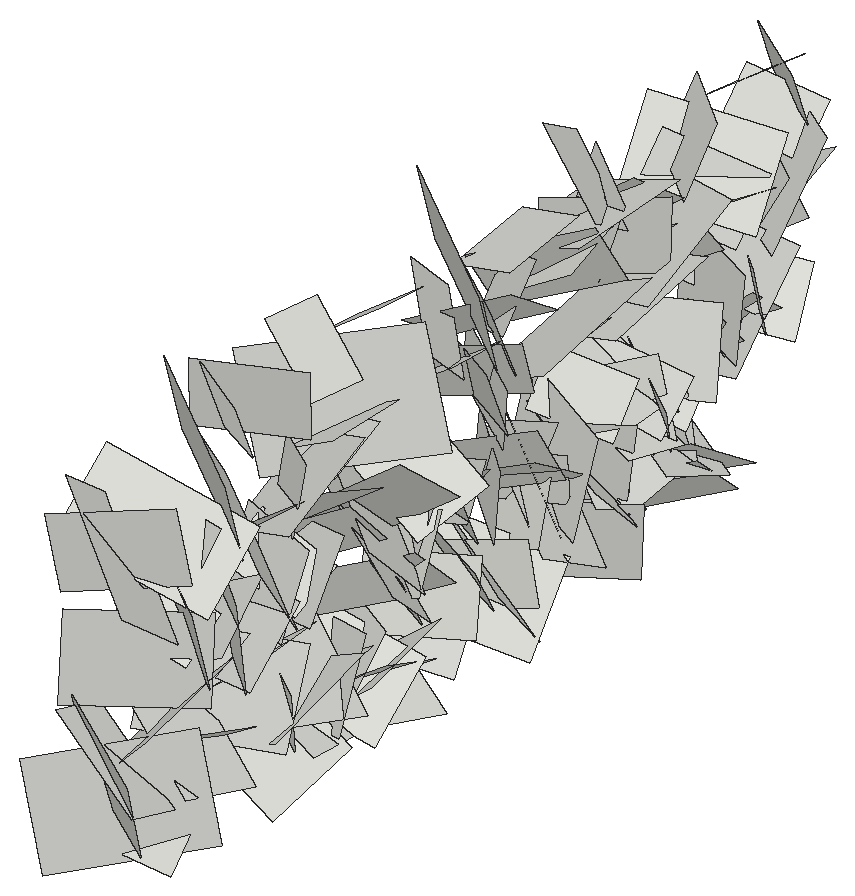
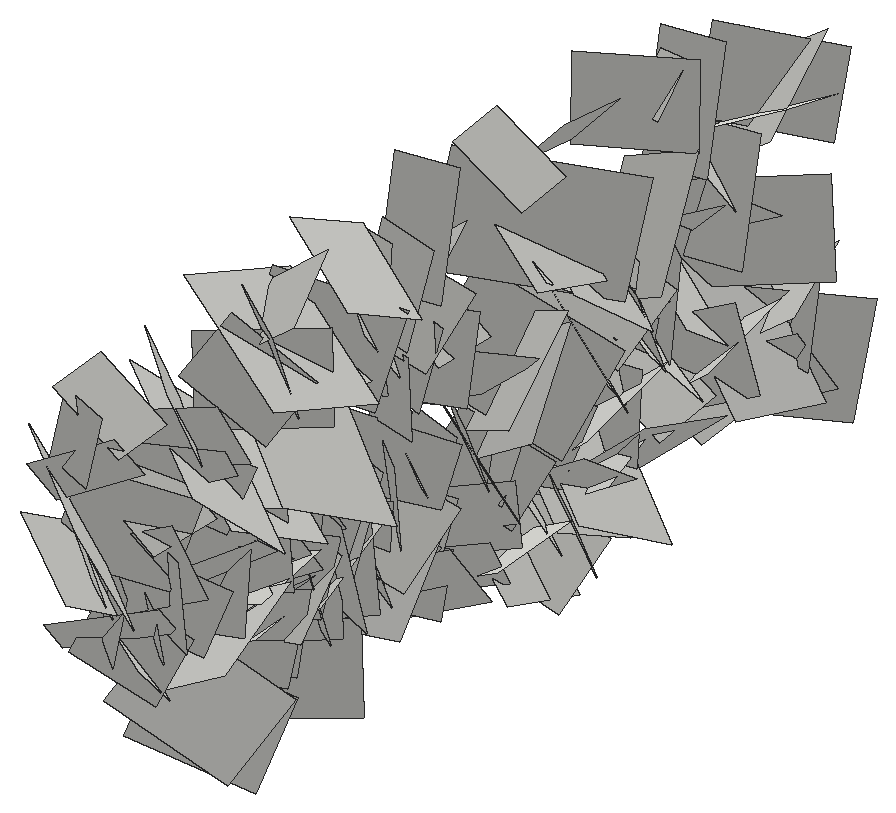
# SketchUp Ruby script. Lengths in inches.
U = 1.inch
M = Sketchup.active_model
def pt(a) = Geom::Point3d.new(a.map { |v| v * U })
def face(e, loops, mat)
  f = e.add_face(loops[0].map { |a| pt(a) })
  loops[1..].each { |l| e.add_face(l.map { |a| pt(a) }).erase! }
  f.material = f.back_material = mat if mat
  f
end
# faces: each face lists its corners as indices into pts; further lists are holes
def faces(e, pts, list, mat = nil) = list.each { |f| face(e, (f[0].is_a?(Array) ? f : [f]).map { |l| l.map { |i| pts[i] } }, mat) }
# xy, xz, yz: faces in a plane at the given z, y or x. An outline is a flat list of corners, or four numbers for a rectangle; further outlines are holes
def ring(l) = l.size == 4 ? [[l[0], l[1]], [l[2], l[1]], [l[2], l[3]], [l[0], l[3]]] : l.each_slice(2).to_a
def flat(e, list, mat, &to3) = list.each { |f| face(e, (f[0].is_a?(Array) ? f : [f]).map { |l| ring(l).map { |u, v| to3.(u, v) } }, mat) }
def xy(e, z, list, mat = nil) = flat(e, list, mat) { |x, y| [x, y, z] }
def xz(e, y, list, mat = nil) = flat(e, list, mat) { |x, z| [x, y, z] }
def yz(e, x, list, mat = nil) = flat(e, list, mat) { |y, z| [x, y, z] }
def lines(e, pts, list) = list.each { |a, b| e.add_line(pt(pts[a]), pt(pts[b])) }
# prism: a flat outline (further loops are holes) pulled along v
def prism(e, loops, v, mat = nil)
  f = face(e, loops, mat); d = Geom::Vector3d.new(v.map { |x| x * U })
  f.pushpull(f.normal.samedirection?(d) ? d.length : -d.length)
end
def box(e, o, s, mat = nil) = prism(e, [[o, [o[0] + s[0], o[1], o[2]], [o[0] + s[0], o[1] + s[1], o[2]], [o[0], o[1] + s[1], o[2]]]], [0, 0, s[2]], mat)
def at(x, y, z, deg = 0) = Geom::Transformation.translation(pt([x, y, z])) * Geom::Transformation.rotation(ORIGIN, Z_AXIS, deg.degrees)
def axes(o, x, y, z) = Geom::Transformation.new([*x, 0, *y, 0, *z, 0, *pt(o).to_a, 1])
def part(name) = M.definitions.add(name)
# library, detail: a bought-in or finely detailed component or shape, given as its bounding box
def library(name, o, s) = part(name).tap { |d| box(d.entities, o, s) }
def detail(e, o, s) = box(e.add_group.entities, o, s)
def put(e, d, t, mat = nil) = e.add_instance(d, t).tap { |i| i.material = mat if mat }
def group(e, t, mat = nil) = e.add_group.tap { |g| g.transformation = t; g.material = mat if mat }.entities
root = M.entities
c1 = part("Component\#6")
p = [[0.01,0,0],[0,3.24,4.54],[4.32,3.24,4.54],[4.33,0,0]]
faces(c1.entities,p,[[0,1,2,3]])
put(root,c1,axes([404.88,126.77,21.87],[0.10992,-0.34124,0.92241],[-0.05569,0.92428,0.34784],[-1.04103,-0.08548,0.07879]))
put(root,c1,axes([400.91,126.29,27.49],[-0.18614,0.86586,-0.34095],[-0.04817,-0.35453,-0.87695],[0.98523,0.14625,-0.10729]))
put(root,c1,axes([404.88,129.02,36.97],[0.03047,0.19902,-0.90037],[-0.05941,-0.89877,-0.20045],[-0.97562,0.06094,-0.01591]))
put(root,c1,axes([404.88,130.54,26.21],[0.16316,0.13144,-1.2549],[0.21583,-1.25022,-0.10597],[-1.31994,-0.18819,-0.17245]))
put(root,c1,axes([404.88,129.15,30.625],[0.089,-0.93417,0.70597],[0.20388,0.70917,0.91554],[-1.22433,0.05019,0.20378]))
put(root,c1,axes([404.88,131.26,22.93],[-0.10206,-0.4663,-0.72841],[-0.02316,-0.73136,0.47108],[-0.91647,0.07041,0.06921]))
put(root,c1,axes([404.88,131.58,31.0625],[-0.07279,0.01987,-1.05868],[0.10279,-1.05633,-0.02611],[-1.11768,-0.09844,0.06655]))
put(root,c1,axes([404.88,127.1,26.99],[0.01407,1.25738,0.35681],[0.29384,0.346,-1.2296],[-1.35392,0.08816,-0.26315]))
put(root,c1,axes([404.88,134.48,33.76],[0.26334,-1.11466,-0.41014],[-0.1173,-0.43892,1.12584],[-1.25351,-0.19309,-0.19152]))
put(root,c1,axes([400.91,129.75,30.06],[0.01937,0.49926,0.36665],[0.0577,0.36409,-0.4985],[0.65405,-0.04691,0.03312]))
put(root,c1,axes([404.88,131.21,27.63],[0.2234,-0.54463,1.08834],[0.02633,1.10624,0.54877],[-1.28976,-0.07175,0.19972]))
put(root,c1,axes([400.91,134.18,33.55],[-0.07538,-0.44425,-0.62436],[0.04133,-0.62833,0.44263],[0.8112,-0.00926,-0.08057]))
put(root,c1,axes([404.88,134.17,21.91],[0.00769,-1.04417,0.30366],[0.13881,0.30229,1.03635],[-1.14428,0.02965,0.12776]))
put(root,c1,axes([400.91,134.6875,22.2],[-0.10426,-0.66856,0.17597],[0.06243,0.169,0.67497],[0.73015,-0.10992,-0.03258]))
put(root,c1,axes([404.88,133.37,32.625],[0.2234,-0.54463,1.08834],[0.02633,1.10624,0.54877],[-1.28976,-0.07175,0.19972]))
put(root,c1,axes([404.88,131.97,28.78],[-0.10091,0.74431,0.53228],[0.01265,0.53611,-0.74754],[-0.96987,-0.07045,-0.06513]))
put(root,c1,axes([404.88,137.68,26.93],[-0.04018,-0.30696,-1.06119],[0.15368,-1.05402,0.2997],[-1.16085,-0.12891,0.07641]))
put(root,c1,axes([404.88,133.57,26.39],[0.0097,-0.16576,1.00827],[0.11893,1.00238,0.16377],[-1.07657,0.10924,0.02717]))
put(root,c1,axes([400.91,135.55,39.48],[0.03347,0.37514,-0.47819],[-0.05412,-0.47551,-0.37641],[0.64197,-0.05964,-0.0068]))
put(root,c1,axes([404.88,133.77,26.39],[0.09062,0.64279,0.71838],[-0.13606,0.72237,-0.63108],[-1.01272,-0.03954,0.14907]))
put(root,c1,axes([404.88,134.64,27.51],[-0.11331,0.92563,-0.03565],[0.09128,-0.0258,-0.92812],[-0.97764,-0.10969,-0.08252]))
put(root,c1,axes([404.88,136.8125,27.97],[0.23976,-0.84366,1.03424],[0.08712,1.0558,0.84327],[-1.41209,-0.07811,0.22763]))
put(root,c1,axes([404.88,137.68,39.44],[-0.12024,0.16456,-0.83242],[-0.12638,-0.83458,-0.14874],[-0.89051,0.09622,0.13351]))
put(root,c1,axes([404.88,140.34,20.98],[-0.05969,-1.08852,-0.33352],[0.17093,-0.33819,1.07653],[-1.19461,0.00599,0.1707]))
put(root,c1,axes([404.88,135.78,27.7],[0.08438,0.31612,0.89331],[-0.15155,0.8902,-0.30228],[-0.99295,-0.109,0.12205]))
put(root,c1,axes([400.91,138.35,27.1],[-0.19626,0.31166,-0.79897],[0.02742,-0.81497,-0.3239],[0.90864,0.09191,-0.1628]))
put(root,c1,axes([400.91,136.92,29.78],[0.03864,0.57092,0.32429],[-0.05823,0.3263,-0.56829],[0.69355,-0.00442,-0.06578]))
put(root,c1,axes([404.88,135.48,23.28],[0.21581,1.04519,0.5846],[0.09636,0.57779,-1.06467],[-1.26577,0.22219,0.01862]))
put(root,c1,axes([400.91,141.16,33.73],[0.01034,-0.20439,-0.70125],[-0.11317,-0.69418,0.20085],[0.76594,-0.09981,0.03914]))
put(root,c1,axes([400.91,137.77,24.11],[-0.1419,0.78136,-0.16109],[0.04598,-0.15597,-0.79258],[0.84441,0.13979,0.01609]))
put(root,c1,axes([404.88,141.41,21.99],[-0.04242,-1.10503,0.33762],[0.18816,0.32793,1.09436],[-1.21025,0.08972,0.15831]))
put(root,c1,axes([404.88,136.3,32.46],[0.17238,0.91042,0.71253],[0.07022,0.71102,-0.92361],[-1.22345,0.16908,0.04738]))
put(root,c1,axes([404.88,137.68,27.62],[-0.00267,0.49736,0.77514],[-0.05686,0.77375,-0.49665],[-0.97459,-0.04651,0.02685]))
put(root,c1,axes([404.88,138.75,33.42],[-0.07987,0.93748,-0.3836],[0.04246,-0.3816,-0.94046],[-1.07286,-0.0849,-0.00867]))
put(root,c1,axes([400.91,143.53,22.21],[-0.15224,-0.84766,-0.36991],[-0.10957,-0.35729,0.85887],[0.97421,-0.17265,0.03879]))
put(root,c1,axes([400.91,139.71,39.61],[0.08624,0.67106,-0.00672],[-0.16105,0.01183,-0.6586],[0.69289,-0.08077,-0.15225]))
put(root,c1,axes([404.88,139.49,21.74],[-0.04906,0.46783,0.90513],[-0.0041,0.90598,-0.46846],[-1.08001,-0.02469,-0.03934]))
put(root,c1,axes([400.91,142.28,27.34],[-0.09885,-0.42767,0.49172],[0.03253,0.4933,0.43487],[0.69002,-0.08452,0.04994]))
put(root,c1,axes([400.91,144.18,33.46],[-0.08879,-0.56105,-0.39599],[0.0694,-0.40364,0.55803],[0.72461,-0.03009,-0.10197]))
put(root,c1,axes([404.88,145.12,23.07],[0.0526,-0.82286,-0.58821],[-0.0059,-0.58914,0.82367],[-1.07215,-0.03713,-0.03339]))
put(root,c1,axes([400.91,144.73,33.27],[-0.16555,-0.76551,-0.15352],[0.02389,-0.16091,0.77946],[0.82725,-0.14855,-0.05323]))
put(root,c1,axes([400.91,142.8,24.59],[-0.06246,-0.31977,0.5346],[0.03506,0.53462,0.32343],[0.65938,-0.05871,0.03344]))
put(root,c1,axes([404.88,145.05,38.54],[0.26561,0.06521,-1.32838],[0.06869,-1.35074,-0.05408],[-1.4081,-0.05359,-0.25321]))
put(root,c1,axes([400.91,145.49,24.46],[-0.14807,-0.32942,-0.64401],[0.00647,-0.65643,0.33444],[0.76675,-0.05808,-0.12719]))
put(root,c1,axes([404.88,142.58,23.75],[-0.11698,0.88265,-0.34817],[0.00423,-0.35009,-0.88876],[-1.00576,-0.10414,0.03675]))
put(root,c1,axes([404.88,143.41,32.67],[0.00295,0.89075,-0.72818],[0.15415,-0.72261,-0.88339],[-1.20976,-0.08991,-0.11434]))
put(root,c1,axes([404.88,145.42,24.52],[0.2647,-0.88765,0.75819],[0.01358,0.77738,0.90589],[-1.23735,-0.18136,0.17214]))
put(root,c1,axes([404.88,141.63,23.18],[0.01995,1.00092,0.30572],[0.13829,0.30114,-0.99396],[-1.10071,0.05598,-0.11933]))
put(root,c1,axes([400.91,145.72,37.21],[0.0202,-0.65006,0.07365],[-0.02062,0.07308,0.65011],[0.69316,0.02112,0.01719]))
put(root,c1,axes([404.88,145.04,25.97],[0.0145,-0.85349,0.83598],[0.13626,0.83223,0.84756],[-1.25903,0.08024,0.10136]))
put(root,c1,axes([404.88,146.5,19.86],[-0.14062,-0.87102,0.18651],[-0.03259,0.19294,0.87915],[-0.94365,0.12313,-0.05815]))
put(root,c1,axes([400.91,145.6,27.28],[0.00806,0.29423,-0.56577],[0.12293,-0.55701,-0.28812],[0.6647,0.09945,0.06014]))
put(root,c1,axes([400.91,146.3,23.53],[-0.0913,-0.50535,0.50896],[0.05568,0.5068,0.51209],[0.75823,-0.09807,0.02368]))
put(root,c1,axes([404.88,144.65,25.96],[-0.15377,0.53431,0.65108],[-0.06081,0.65286,-0.54856],[-0.89071,-0.13681,-0.07495]))
put(root,c1,axes([404.88,149.17,29.19],[-0.22051,-0.77582,-0.34275],[0.07369,-0.36732,0.78924],[-0.89602,0.16072,0.14925]))
put(root,c1,axes([400.91,149.12,29.1],[-0.10824,-0.19319,-0.65872],[-0.02698,-0.66445,0.19881],[0.72715,-0.05341,-0.09068]))
put(root,c1,axes([400.91,145.7,22.51],[-0.08358,0.19729,0.79599],[-0.0899,0.79341,-0.20506],[0.86462,0.10156,0.05562]))
put(root,c1,axes([400.91,146.45,21.25],[-0.00375,0.2874,0.54008],[0.0654,0.5375,-0.28562],[0.64519,-0.05282,0.03209]))
put(root,c1,axes([400.91,149.08,38.35],[0.0057,0.54335,-0.52891],[-0.23788,-0.50408,-0.52014],[0.76776,-0.16022,-0.15723]))
put(root,c1,axes([400.91,150.81,32.67],[-0.03105,-0.70657,0.01303],[0.00041,0.01303,0.70717],[0.74909,-0.02929,0.00015]))
put(root,c1,axes([400.91,149.71,29.1],[0.04042,0.22115,-0.567],[0.10046,-0.56334,-0.21335],[0.63725,0.07479,0.0696]))
put(root,c1,axes([400.91,149.63,26.39],[-0.05575,0.3601,-0.58557],[0.15834,-0.56726,-0.36226],[0.71127,0.15451,0.03475]))
put(root,c1,axes([404.88,149.65,34.23],[0.2234,-0.54463,1.08834],[0.02633,1.10624,0.54877],[-1.28976,-0.07175,0.19972]))
put(root,c1,axes([400.91,151.89,27.92],[0.07457,-0.37507,-0.49968],[-0.035,-0.50437,0.37394],[0.66135,0.0156,0.07613]))
put(root,c1,axes([404.88,150.4,30.92],[-0.04252,-0.27759,0.76161],[-0.13298,0.75548,0.26875],[-0.84891,-0.10444,-0.08025]))
put(root,c1,axes([404.88,151.25,34.8],[-0.16779,0.3958,-0.75565],[-0.05631,-0.77163,-0.39305],[-0.90246,-0.02545,0.16502]))
put(root,c1,axes([404.88,150.92,33.45],[0.01124,-0.40239,0.85237],[-0.02564,0.85203,0.40253],[-0.99881,-0.0264,-0.00074]))
put(root,c1,axes([404.88,150.56,37.37],[-0.01495,0.72639,-0.4873],[-0.06872,-0.48689,-0.7239],[-0.92463,0.02444,0.06168]))
put(root,c1,axes([400.91,150.69,21.46],[-0.08617,-0.06424,0.73191],[0.1147,0.7273,0.07585],[0.77031,-0.11548,0.07058]))
put(root,c1,axes([404.88,154.4,23.625],[0.0407,-0.65785,-0.83395],[-0.03781,-0.83482,0.65689],[-1.12528,0.00426,-0.05223]))
put(root,c1,axes([400.91,152.7,33.94],[-0.15183,0.13661,-0.74127],[0.04087,-0.75222,-0.14607],[0.79793,0.06452,-0.13357]))
put(root,c1,axes([400.91,153.52,29.46],[-0.08102,0.00764,-0.81457],[-0.10707,-0.81193,0.00187],[0.85682,-0.10074,-0.07679]))
put(root,c1,axes([404.88,152.42,20.54],[0.05004,-0.6691,0.77955],[-0.05919,0.77755,0.67076],[-1.08735,-0.07312,-0.00064]))
put(root,c1,axes([404.88,152.27,30.34],[-0.04267,0.47891,-0.74389],[-0.05776,-0.74459,-0.47642],[-0.93603,0.02411,0.06331]))
put(root,c1,axes([400.91,155.3,36.05],[-0.02231,-0.46484,-0.62566],[-0.10069,-0.6197,0.4636],[0.82005,-0.08874,0.0399]))
put(root,c1,axes([404.88,152.14,28.92],[-0.00837,0.82237,-0.50147],[-0.16225,-0.49618,-0.8113],[-1.00803,0.07304,0.13474]))
put(root,c1,axes([400.91,156.34,37.48],[-0.20366,-0.78098,-0.33642],[0.07649,-0.35863,0.79133],[0.89812,-0.14656,-0.14368]))
put(root,c1,axes([404.88,152.31,24.83],[-0.14132,0.38772,0.61473],[-0.11706,0.60692,-0.40674],[-0.76145,-0.16526,-0.05156]))
put(root,c1,axes([400.91,153.82,25.23],[0.04726,-0.11023,0.59197],[0.093,0.58845,0.10297],[0.63147,-0.07841,-0.05947]))
put(root,c1,axes([404.88,153.79,24.7],[0.00565,-0.43188,0.90191],[0.04751,0.90112,0.43124],[-1.05892,0.03812,0.02416]))
put(root,c1,axes([404.88,156.72,22.08],[0.00521,-0.94479,0.50901],[0.17637,0.50353,0.93301],[-1.12382,0.07464,0.14878]))
put(root,c1,axes([404.88,155.99,38.05],[-0.0315,0.52335,-0.79271],[0.01447,-0.79278,-0.52391],[-1.00678,-0.02777,0.01727]))
put(root,c1,axes([404.88,154.59,24.16],[0.1724,0.15274,1.09758],[-0.17194,1.10067,-0.12914],[-1.16199,-0.14021,0.18195]))
put(root,c1,axes([404.88,154.45,36.57],[-0.07713,0.81709,0.22722],[-0.03645,0.22503,-0.82021],[-0.89825,-0.07929,0.01378]))
put(root,c1,axes([400.91,158.01,30.39],[0.08038,-0.60995,0.00551],[-0.02253,0.00291,0.6143],[0.64618,0.07598,0.02073]))
put(root,c1,axes([404.88,152.65,32.7],[0.31384,1.21799,0.62272],[0.13011,0.61092,-1.25326],[-1.44417,0.31973,0.02242]))
put(root,c1,axes([404.88,158.66,27.8],[-0.19419,0.10037,-0.91545],[0.10975,-0.92523,-0.12216],[-0.97001,-0.12478,0.16945]))
put(root,c1,axes([400.91,158.73,27.09],[-0.13155,-0.14233,-0.74779],[-0.00006,-0.75766,0.14422],[0.80689,-0.02326,-0.12191]))
put(root,c1,axes([404.88,159.15,23.91],[-0.14407,0.13595,-0.90237],[0.02833,-0.91134,-0.14133],[-0.9669,-0.04696,0.13032]))
put(root,c1,axes([400.91,156.49,28.09],[0.01227,0.36562,0.53928],[0.0952,0.53332,-0.36351],[0.68404,-0.08079,0.04092]))
put(root,c1,axes([400.91,156.65,23.33],[0.01341,0.01203,0.69899],[-0.10657,0.69187,-0.01009],[0.73333,0.10033,-0.01425]))
put(root,c1,axes([404.88,158.65,23.12],[0.03,-0.65446,0.65644],[-0.11713,0.64968,0.65248],[-0.97555,-0.09812,-0.05816]))
put(root,c1,axes([404.88,154.96,37.56],[0.27688,1.1515,0.31839],[-0.11464,0.34737,-1.16756],[-1.26119,0.22122,0.17603]))
put(root,c1,axes([400.91,157.59,40.82],[-0.16311,0.68993,-0.43022],[-0.09586,-0.44966,-0.68876],[0.85651,0.08106,-0.15901]))
put(root,c1,axes([400.91,161,38.46],[-0.19651,-0.13504,-0.81499],[-0.03185,-0.8336,0.14496],[0.87508,-0.06067,-0.17773]))
put(root,c1,axes([400.91,158.75,26.14],[0.12859,0.59437,-0.23179],[-0.06253,-0.22448,-0.60651],[0.67335,-0.13435,-0.01206]))
put(root,c1,axes([404.88,160.9375,37.33],[-0.13153,0.12633,-0.90974],[0.10231,-0.91113,-0.13969],[-0.96819,-0.11344,0.10882]))
put(root,c1,axes([400.91,158.03,24.73],[-0.19324,-0.05037,0.89121],[-0.15909,0.89838,0.02008],[0.93272,0.1428,0.18806]))
put(root,c1,axes([400.91,158.35,30.49],[-0.08461,0.81055,-0.03501],[-0.12527,-0.04642,-0.80528],[0.85081,0.07377,-0.12204]))
put(root,c1,axes([404.88,161.79,25.53],[-0.01152,-0.82607,0.19056],[-0.15176,0.18963,0.81386],[-0.88572,-0.02175,-0.14193]))
put(root,c1,axes([404.88,162.32,28.44],[-0.12821,-0.42216,-0.69512],[0.01339,-0.70366,0.42514],[-0.86197,0.05186,0.11]))
put(root,c1,axes([400.91,158.39,26.84],[-0.02686,0.84806,0.10272],[-0.17857,0.09579,-0.83237],[0.88773,0.04493,-0.16432]))
put(root,c1,axes([400.91,161.42,33.85],[-0.12931,-0.58697,0.4315],[-0.06321,0.44408,0.58723],[0.76963,-0.06214,0.12073]))
put(root,c1,axes([404.88,157.3125,32.29],[0.25179,1.05256,0.51222],[-0.06429,0.53303,-1.06718],[-1.23914,0.18623,0.15945]))
put(root,c1,axes([400.91,160.06,22.6],[-0.02839,-0.24478,0.77995],[-0.15528,0.76918,0.23637],[0.85248,0.13195,0.06903]))
put(root,c1,axes([400.91,159.46,22.85],[-0.09982,-0.0635,0.89488],[-0.1784,0.88507,0.04509],[0.93408,0.16225,0.10424]))
put(root,c1,axes([400.91,162.33,29.83],[-0.22776,0.38392,-0.75072],[0.01782,-0.77261,-0.39993],[0.89361,0.11326,-0.18337]))
put(root,c1,axes([404.88,164.2,31.01],[0.06613,-0.18181,-0.96198],[-0.02897,-0.96387,0.1804],[-1.03734,0.01533,-0.06637]))
put(root,c1,axes([400.91,159.67,28.14],[-0.12868,0.67272,0.52517],[-0.08613,0.51893,-0.68352],[0.90053,0.14576,0.00967]))
put(root,c1,axes([404.88,162.55,24.47],[-0.08094,0.6993,-0.63815],[-0.06519,-0.64254,-0.69674],[-1.00139,-0.01469,0.09694]))
put(root,c1,axes([404.88,164.67,22.86],[0.07455,-1.03669,0.46758],[-0.01691,0.46753,1.03897],[-1.20537,-0.07068,0.01434]))
put(root,c1,axes([404.88,159.15,32.85],[0.28722,0.93511,0.86971],[0.00467,0.88838,-0.95656],[-1.35365,0.20148,0.18123]))
put(root,c1,axes([404.88,162.15,25.43],[0.09766,0.84172,-0.54191],[-0.18116,-0.52299,-0.84139],[-1.04557,0.16923,0.09516]))
put(root,c1,axes([400.91,163.79,31.02],[-0.0186,-0.39942,0.51021],[-0.04828,0.50989,0.39761],[0.68514,0.02509,0.04187]))
put(root,c1,axes([400.91,165.16,26.22],[0.00662,-0.41647,0.48084],[-0.04981,0.47925,0.41571],[0.67246,0.0396,0.02606]))
put(root,c1,axes([400.91,167.47,38.84],[-0.19203,-0.25676,-0.78485],[-0.09527,-0.79261,0.28005],[0.87013,-0.14344,-0.14255]))
put(root,c1,axes([404.88,167.29,35.58],[-0.17595,-0.29467,-0.74084],[-0.05215,-0.7515,0.30993],[-0.84352,0.10793,0.13537]))
put(root,c1,axes([404.88,168.37,37.02],[0.06582,-0.55881,-0.84289],[-0.17414,-0.83883,0.54402],[-1.05774,0.10333,-0.14201]))
put(root,c1,axes([404.88,165.04,27.71],[0.04822,0.07219,0.94774],[-0.14201,0.93984,-0.06516],[-0.99746,-0.13032,0.05509]))
put(root,c1,axes([400.91,168.23,31.98],[-0.11552,-0.73847,0.10601],[0.00435,0.10653,0.74638],[0.79079,-0.10846,0.01138]))
put(root,c1,axes([400.91,168.24,29.62],[-0.00844,-0.1319,-0.59476],[-0.00779,-0.59475,0.132],[0.64572,-0.0089,-0.00618]))
put(root,c1,axes([400.91,169.17,27.35],[0.00515,-0.4485,-0.48712],[0.04455,-0.48594,0.44784],[0.70046,0.0342,-0.02491]))
put(root,c1,axes([404.88,169.13,31.47],[-0.22896,-0.22184,-0.76377],[-0.12794,-0.77313,0.25869],[-0.83329,0.17965,0.17014]))
put(root,c1,axes([400.91,168.14,25.37],[-0.00005,-0.54267,0.44601],[-0.16088,0.43548,0.52984],[0.72699,0.09633,0.11728]))
put(root,c1,axes([400.91,167.3,30.05],[-0.09755,-0.36279,0.79394],[-0.2327,0.7823,0.33203],[0.89554,0.16375,0.17276]))
put(root,c1,axes([400.91,169.92,30.86],[0.08798,0.07784,-0.70174],[-0.08853,-0.70052,-0.08758],[0.74315,-0.09267,0.07264]))
put(root,c1,axes([400.91,170.38,37.22],[-0.01844,-0.65259,0.06973],[-0.0154,0.07012,0.65262],[0.69551,-0.01575,0.0163]))
put(root,c1,axes([400.91,166.74,28.03],[-0.20581,0.5378,0.53941],[0.0447,0.5634,-0.54654],[0.80617,0.10606,0.16802]))
put(root,c1,axes([400.91,171.91,32.4],[0.07209,-0.36069,-0.54144],[-0.07785,-0.54516,0.35394],[0.6852,-0.024,0.09718]))
put(root,c1,axes([400.91,168.82,35.84],[0.04533,0.37689,0.51175],[-0.01637,0.51337,-0.3768],[0.67349,-0.01289,-0.04361]))
put(root,c1,axes([404.88,167.34,31.77],[0.2501,0.51374,1.1242],[0.05799,1.13903,-0.532],[-1.3089,0.14863,0.19123]))
put(root,c1,axes([400.91,171.42,39.46],[0.01769,0.21401,-0.61924],[0.03571,-0.6189,-0.21298],[0.69357,0.02641,0.02676]))
put(root,c1,axes([400.91,173.67,32.24],[-0.05341,-0.65994,-0.37026],[-0.06447,-0.36634,0.66124],[0.79951,-0.07362,0.02859]))
